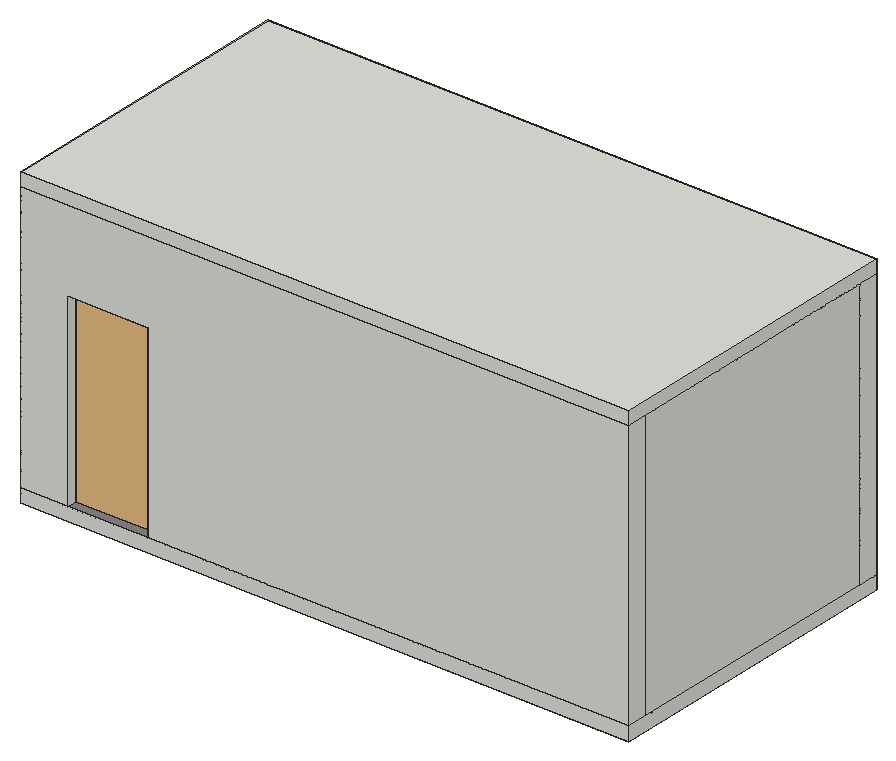
# SketchUp Ruby script. Lengths in inches.
U = 1.inch
M = Sketchup.active_model
def pt(a) = Geom::Point3d.new(a.map { |v| v * U })
def face(e, loops, mat)
  f = e.add_face(loops[0].map { |a| pt(a) })
  loops[1..].each { |l| e.add_face(l.map { |a| pt(a) }).erase! }
  f.material = f.back_material = mat if mat
  f
end
# faces: each face lists its corners as indices into pts; further lists are holes
def faces(e, pts, list, mat = nil) = list.each { |f| face(e, (f[0].is_a?(Array) ? f : [f]).map { |l| l.map { |i| pts[i] } }, mat) }
# xy, xz, yz: faces in a plane at the given z, y or x. An outline is a flat list of corners, or four numbers for a rectangle; further outlines are holes
def ring(l) = l.size == 4 ? [[l[0], l[1]], [l[2], l[1]], [l[2], l[3]], [l[0], l[3]]] : l.each_slice(2).to_a
def flat(e, list, mat, &to3) = list.each { |f| face(e, (f[0].is_a?(Array) ? f : [f]).map { |l| ring(l).map { |u, v| to3.(u, v) } }, mat) }
def xy(e, z, list, mat = nil) = flat(e, list, mat) { |x, y| [x, y, z] }
def xz(e, y, list, mat = nil) = flat(e, list, mat) { |x, z| [x, y, z] }
def yz(e, x, list, mat = nil) = flat(e, list, mat) { |y, z| [x, y, z] }
def lines(e, pts, list) = list.each { |a, b| e.add_line(pt(pts[a]), pt(pts[b])) }
# prism: a flat outline (further loops are holes) pulled along v
def prism(e, loops, v, mat = nil)
  f = face(e, loops, mat); d = Geom::Vector3d.new(v.map { |x| x * U })
  f.pushpull(f.normal.samedirection?(d) ? d.length : -d.length)
end
def box(e, o, s, mat = nil) = prism(e, [[o, [o[0] + s[0], o[1], o[2]], [o[0] + s[0], o[1] + s[1], o[2]], [o[0], o[1] + s[1], o[2]]]], [0, 0, s[2]], mat)
def at(x, y, z, deg = 0) = Geom::Transformation.translation(pt([x, y, z])) * Geom::Transformation.rotation(ORIGIN, Z_AXIS, deg.degrees)
def axes(o, x, y, z) = Geom::Transformation.new([*x, 0, *y, 0, *z, 0, *pt(o).to_a, 1])
def part(name) = M.definitions.add(name)
# library, detail: a bought-in or finely detailed component or shape, given as its bounding box
def library(name, o, s) = part(name).tap { |d| box(d.entities, o, s) }
def detail(e, o, s) = box(e.add_group.entities, o, s)
def put(e, d, t, mat = nil) = e.add_instance(d, t).tap { |i| i.material = mat if mat }
def group(e, t, mat = nil) = e.add_group.tap { |g| g.transformation = t; g.material = mat if mat }.entities
root = M.entities
M.materials.add("Generic\#1").color = [255, 244, 244]
M.materials.add("Generic\#2").color = [136, 130, 130]
M.materials.add("Tiles Simple 03 100cm").color = [137, 132, 131]
M.materials.add("Wine2").color = [0, 0, 0]
M.materials["Wine2"].alpha = 0
M.materials.add("[0130_Gainsboro]").color = [39, 45, 50]
M.materials.add("[Color F08]").color = [51, 102, 0]
M.materials.add("[Color K01]").color = [128, 97, 74]
M.materials.add("[Color M07]").color = [58, 58, 58]
M.materials.add("[Wood Veneer 01]").color = [120, 70, 37]
c1 = library("Tlon Light 450 Ceiling 152 006",[-8.86,-8.86,-3.78],[17.72,17.72,3.56])
c2 = part("Framed panel")
xy(c2.entities,0,[[0,-0.98,43.07,0],[0,0,43.07,1.4]],"[0130_Gainsboro]")
xy(c2.entities,0.3,[[0.3,-1.43,42.77,-0.98]],"[0130_Gainsboro]")
xy(c2.entities,2.95,[[2.95,-1.43,40.12,-0.63],[2.95,-0.63,40.12,0],[2.95,0,40.12,0.64],[2.95,0.64,40.12,1.4]],"[0130_Gainsboro]")
xy(c2.entities,3.54,[[3.54,-0.63,39.53,0],[3.54,0,39.53,0.64]],"[0130_Gainsboro]")
xy(c2.entities,111.8125,[[3.54,-0.63,39.53,0],[3.54,0,39.53,0.64]],"[0130_Gainsboro]")
xy(c2.entities,112.4,[[2.95,-1.43,40.12,-0.63],[2.95,-0.63,40.12,0],[2.95,0,40.12,0.64],[2.95,0.64,40.12,1.4]],"[0130_Gainsboro]")
xy(c2.entities,115.05,[[0.3,-1.43,42.77,-0.98]],"[0130_Gainsboro]")
xy(c2.entities,115.35,[[0,-0.98,43.07,0],[0,0,43.07,1.4]],"[0130_Gainsboro]")
xz(c2.entities,-1.43,[[[0.3,0.3,42.77,115.05],[2.95,2.95,40.12,112.4]]],"[0130_Gainsboro]")
xz(c2.entities,-0.98,[[[0,0,43.07,115.35],[0.3,0.3,42.77,115.05]]],"[0130_Gainsboro]")
xz(c2.entities,-0.63,[[[2.95,2.95,40.12,112.4],[3.54,3.54,39.53,111.8125]]],"[0130_Gainsboro]")
xz(c2.entities,0,[[3.54,3.54,39.53,111.8125]],"Wine2")
xz(c2.entities,0,[[[0,0,43.07,115.35],[2.95,2.95,40.12,112.4]],[[2.95,2.95,40.12,112.4],[3.54,3.54,39.53,111.8125]]],"[0130_Gainsboro]")
xz(c2.entities,0.64,[[[2.95,2.95,40.12,112.4],[3.54,3.54,39.53,111.8125]]],"[0130_Gainsboro]")
xz(c2.entities,1.4,[[[0,0,43.07,115.35],[2.95,2.95,40.12,112.4]]],"[0130_Gainsboro]")
yz(c2.entities,0,[[-0.98,0,0,115.35],[0,0,1.4,115.35]],"[0130_Gainsboro]")
yz(c2.entities,0.3,[[-1.43,0.3,-0.98,115.05]],"[0130_Gainsboro]")
yz(c2.entities,2.95,[[-1.43,2.95,-0.63,112.4],[-0.63,2.95,0,112.4],[0,2.95,0.64,112.4],[0.64,2.95,1.4,112.4]],"[0130_Gainsboro]")
yz(c2.entities,3.54,[[-0.63,3.54,0,111.8125],[0,3.54,0.64,111.8125]],"[0130_Gainsboro]")
yz(c2.entities,39.53,[[-0.63,3.54,0,111.8125],[0,3.54,0.64,111.8125]],"[0130_Gainsboro]")
yz(c2.entities,40.12,[[-1.43,2.95,-0.63,112.4],[-0.63,2.95,0,112.4],[0,2.95,0.64,112.4],[0.64,2.95,1.4,112.4]],"[0130_Gainsboro]")
yz(c2.entities,42.77,[[-1.43,0.3,-0.98,115.05]],"[0130_Gainsboro]")
yz(c2.entities,43.07,[[-0.98,0,0,115.35],[0,0,1.4,115.35]],"[0130_Gainsboro]")
c3 = part("Framed panel assembly")
put(c3.entities,c2,axes([90.57,1.43,0],[1.05148,0,0],[0,1,0],[0,0,1]))
put(c3.entities,c2,axes([0,1.43,0],[1.05148,0,0],[0,1,0],[0,0,1]))
put(c3.entities,c2,axes([45.29,1.43,0],[1.05148,0,0],[0,1,0],[0,0,1]))
c4 = library("12",[-59.59,-13.96,0.05],[132.77,19.46,130.21])
c5 = library("porta 4",[0.2,-5.42,1.33],[46.55,4.72,83.21])
c6 = library("TV Stand 144 005",[-36.8,-10.43,-0.15],[73.6,20.86,18.87])
c7 = library("Decoration 111 063",[-2.51,-1.28,-0.03],[5.02,2.53,10.66])
c8 = library("Vase Roses Red 63-02",[-2.39,-2.73,0.01],[6.39,5.25,18.18])
c9 = library("Decorative Deer 209 004",[-1.58,-4.16,0],[3.36,7.25,10.63])
c10 = library("TV Flatscreen 001",[-21.34,-8.66,-0.01],[42.68,15.88,27.55])
c11 = library("Tree Of Life Wall Art",[0,-2.17,0],[76.8125,2.17,76.8125])
c12 = library("Potted plant",[-1.15,-1.29,0],[7.65,7.78,5.89])
c13 = library("Chloe Sofa",[-57.875,-21.08,0],[115.75,42.01,35.79])
c14 = library("Vavel Meeting",[-46.89,-19.24,-0.01],[93.78,38.48,29.4])
c15 = library("Vase 007",[-9.22,-3.28,0],[11.85,5.91,21.89])
c16 = library("Armillary Sphere 37-31",[-7.11,-7.1,0],[14.21,14.18,18.13])
c17 = library("Aroma Diffuser 274 006",[-1.2,-1.19,-0.07],[2.39,2.37,8.4])
c18 = library("Carpet 274 003",[-39.19,-39.17,0],[78.4,78.37,0.4])
c19 = library("Apple 73-11",[-5.39,-5.39,0],[10.78,10.78,8.98])
c20 = library("Books 193 006",[-5.22,-3.55,0],[10.44,7.83,2.69])
c21 = library("ceiling fan",[14.63,0,0.68],[45.1,74.31,31.88])
c22 = part("fan")
p = [[217.527,-902.72,540.318],[217.529,-902.72,540.318],[217.529,-902.72,541.354],[217.527,-902.72,541.354]]
lines(c22.entities,p,[[0,1],[2,3]])
put(c22.entities,c21,at(256.45,-350.9,679.41))
c23 = library("Group\#2",[-0.5,0,0.5],[103.99,27.6,2])
c24 = library("Group\#4",[-0.5,-0.5,0],[103.99,10.6875,2])
c25 = library("Group\#5",[-0.5,-0.5,0],[150.41,81.41,2])
c26 = library("Group\#8",[0,0,0],[11.8125,120,116])
c27 = library("Group\#16",[-0.5,-0.5,-0.1],[1.5,51,0.2])
c28 = library("Group\#17",[-0.5,-0.5,0],[1.5,1,93.9375])
c29 = library("Group\#18",[-0.5,-0.5,0],[1.5,1,93.9375])
c30 = library("Group\#19",[-0.5,-0.5,-0.1],[1.5,51,0.2])
xy(root,-6,[[0,0,270.9375,138]])
xy(root,0,[[0,0,21,0,21,9,9,9,9,129,270.9375,129,270.9375,138,0,138],[57,0,270.9375,9]])
xy(root,0,[[21,0,57,0,57,9,270.9375,9,270.9375,129,9,129,9,32.0625,20.8125,32.0625,20.8125,9,21,9]],"Tiles Simple 03 100cm")
xy(root,4.46,[[18.45,129,187.89,138]])
xy(root,22.0625,[[9.5,44.37,9.9,94.37]])
xy(root,52.39,[[85.32,9,126.94,10.0625]],"[Color M07]")
xy(root,54.875,[[87.81,9.375,124.46,10.0625]],"[Color M07]")
xy(root,84,[[21,0,57,9]])
xy(root,88.84,[[18.45,129,187.89,138]])
xy(root,102.34,[[87.81,9.375,124.46,10.0625]],"[Color M07]")
xy(root,104.82,[[85.32,9,126.94,10.0625]],"[Color M07]")
xy(root,116,[[[9,9,198,129],[30.8,30.8,176.2,107.2],[9.5,44.37,9.9,94.37]],[9.5,44.37,9.9,94.37]],"Generic\#2")
xy(root,116,[[45.6,45.6,45.6,63.5,54,63.5,54,54,153,54,153,63.5,161.4,63.5,161.4,45.6],[45.6,76.31,45.6,92.4,161.4,92.4,161.4,76.31,153,76.31,153,84,54,84,54,76.31]],"[Wood Veneer 01]")
xy(root,118,[[28.8,28.8,30.8,107.2],[30.8,28.8,178.2,30.8],[176.2,30.8,178.2,107.2],[52,52,155,54],[52,54,54,63.5],
  [153,54,155,63.5],[52,76.31,54,86],[153,76.31,155,84],[54,84,155,86],[28.8,107.2,178.2,109.2]])
xy(root,120,[[0,0,0,138,270.9375,138,270.9375,129,9,129,9,9,270.9375,9,270.9375,0],[[9,9,198,129],[28.8,28.8,178.2,109.2]],[198,9,270.9375,129]])
xy(root,120,[[[28.8,28.8,178.2,109.2],[45.6,45.6,161.4,45.6,161.4,63.5,155,63.5,155,52,52,52,52,63.5,45.6,63.5],[45.6,76.31,52,76.31,52,86,155,86,155,76.31,161.4,76.31,161.4,92.4,45.6,92.4],[96.37,61.16,97.05,61.17,97.73,61.22,98.41,61.33,99.08,61.49,99.73,61.71,100.36,61.97,100.97,62.28,101.55,62.64,102.11,63.05,102.625,63.49,103.11,63.98,103.55,64.5,103.95,65.06,104.31,65.64,104.62,66.25,104.88,66.89,105.09,67.54,105.25,68.21,105.35,68.88,105.4,69.57,105.4,70.25,105.35,70.93,105.24,71.61,105.08,72.28,104.86,72.93,104.6,73.56,104.29,74.17,103.93,74.75,103.52,75.31,103.08,75.83,102.59,76.31,102.07,76.75,101.51,77.15,100.93,77.51,100.32,77.82,99.68,78.08,99.03,78.29,98.36,78.45,97.6875,78.55,97,78.61,96.32,78.6,95.63,78.55,94.96,78.4375,94.29,78.28,93.64,78.0625,93.01,77.8,92.4,77.49,91.82,77.125,91.26,76.72,90.74,76.28,90.26,75.79,89.82,75.27,89.42,74.71,89.06,74.13,88.75,73.52,88.49,72.88,88.28,72.23,88.12,71.5625,88.02,70.89,87.96,70.2,87.97,69.52,88.02,68.83,88.13,68.16,88.29,67.49,88.51,66.84,88.77,66.21,89.08,65.6,89.44,65.02,89.85,64.46,90.29,63.94,90.78,63.46,91.3,63.02,91.86,62.62,92.44,62.26,93.05,61.95,93.6875,61.69,94.34,61.48,95.01,61.32,95.68,61.22]]],"Generic\#2")
xy(root,126,[[0,0,270.9375,138]])
xz(root,0,[[0,-6,270.9375,0],[0,0,21,0,21,84,57,84,57,0,270.9375,0,270.9375,120,0,120],[0,120,270.9375,126]])
xz(root,9,[[85.32,52.39,126.94,104.82],[9,116,198,120],[198,116,270.9375,120]])
xz(root,9,[[[9,0,9,116,270.9375,116,270.9375,0,57,0,57,84,21,84,21,0],[85.32,52.39,126.94,104.82]]],"Generic\#2")
xz(root,9.375,[[87.81,54.875,124.46,102.34]],"[Color K01]")
xz(root,10.0625,[[[85.32,52.39,126.94,104.82],[87.81,54.875,124.46,102.34]]],"[Color M07]")
xz(root,30.8,[[30.8,116,176.2,118]],"Generic\#2")
xz(root,44.37,[[9.5,22.0625,9.9,116]])
xz(root,45.6,[[45.6,116,161.4,120]],"[Wood Veneer 01]")
xz(root,54,[[54,116,153,118]],"[Wood Veneer 01]")
xz(root,63.5,[[45.6,116,45.6,120,52,120,52,118,54,118,54,116],[153,116,153,118,155,118,155,120,161.4,120,161.4,116]],"[Wood Veneer 01]")
xz(root,76.31,[[45.6,116,54,116,54,118,52,118,52,120,45.6,120],[153,116,161.4,116,161.4,120,155,120,155,118,153,118]],"[Wood Veneer 01]")
xz(root,84,[[54,116,153,118]],"[Wood Veneer 01]")
xz(root,92.4,[[45.6,116,161.4,120]],"[Wood Veneer 01]")
xz(root,94.37,[[9.5,22.0625,9.9,116]])
xz(root,107.2,[[30.8,116,176.2,118]],"Generic\#2")
xz(root,129,[[9,116,198,120],[198,116,270.9375,120]])
xz(root,129,[[[9,0,270.9375,116],[18.45,4.46,187.89,88.84]]],"Generic\#2")
xz(root,138,[[0,-6,270.9375,0],[[0,0,270.9375,120],[18.45,4.46,187.89,88.84]],[0,120,270.9375,126]])
yz(root,0,[[0,-6,138,0],[0,0,138,120],[0,120,138,126]])
yz(root,9,[[[44.37,22.0625,94.37,116],[70.2,57.86,71.66,57.9375,73.11,58.12,74.55,58.4,75.96,58.78,77.34,59.26,78.6875,59.84,79.99,60.51,81.24,61.26,82.4375,62.1,83.57,63.03,84.64,64.03,85.64,65.1,86.55,66.24,87.39,67.4375,88.14,68.69,88.8,70,89.37,71.35,89.84,72.73,90.22,74.14,90.5,75.58,90.67,77.03,90.74,78.49,90.71,79.96,90.58,81.41,90.35,82.86,90.02,84.28,89.59,85.68,89.0625,87.04,88.44,88.37,87.73,89.65,86.93,90.87,86.05,92.04,85.08,93.14,84.05,94.17,82.94,95.13,81.77,96.01,80.54,96.8,79.26,97.51,77.93,98.12,76.57,98.64,75.17,99.07,73.74,99.39,72.3,99.62,70.84,99.74,69.375,99.77,67.92,99.6875,66.46,99.5,65.03,99.22,63.62,98.84,62.23,98.36,60.89,97.79,59.59,97.12,58.33,96.36,57.14,95.52,56,94.6,54.9375,93.6,53.94,92.53,53.02,91.39,52.1875,90.1875,51.4375,88.93,50.77,87.63,50.21,86.28,49.73,84.9,49.36,83.48,49.08,82.05,48.91,80.59,48.83,79.13,48.86,77.67,48.99,76.21,49.22,74.77,49.56,73.34,49.99,71.95,50.51,70.58,51.14,69.26,51.85,67.98,52.65,66.75,53.53,65.59,54.49,64.49,55.53,63.45,56.64,62.5,57.81,61.62,59.03,60.82,60.32,60.12,61.64,59.5,63.01,58.98,64.41,58.56,65.83,58.23,67.28,58.01,68.74,57.88]],[9,116,129,120]])
yz(root,9,[[9,0,129,0,129,116,94.37,116,94.37,22.0625,44.37,22.0625,44.37,116,9,116]],"Generic\#2")
yz(root,9.5,[[[44.37,22.0625,94.37,116],[70.2,57.86,71.66,57.9375,73.11,58.12,74.55,58.4,75.96,58.78,77.34,59.26,78.6875,59.84,79.99,60.51,81.24,61.26,82.4375,62.1,83.57,63.03,84.64,64.03,85.64,65.1,86.55,66.24,87.39,67.4375,88.14,68.69,88.8,70,89.37,71.35,89.84,72.73,90.22,74.14,90.5,75.58,90.67,77.03,90.74,78.49,90.71,79.96,90.58,81.41,90.35,82.86,90.02,84.28,89.59,85.68,89.0625,87.04,88.44,88.37,87.73,89.65,86.93,90.87,86.05,92.04,85.08,93.14,84.05,94.17,82.94,95.13,81.77,96.01,80.54,96.8,79.26,97.51,77.93,98.12,76.57,98.64,75.17,99.07,73.74,99.39,72.3,99.62,70.84,99.74,69.375,99.77,67.92,99.6875,66.46,99.5,65.03,99.22,63.62,98.84,62.23,98.36,60.89,97.79,59.59,97.12,58.33,96.36,57.14,95.52,56,94.6,54.9375,93.6,53.94,92.53,53.02,91.39,52.1875,90.1875,51.4375,88.93,50.77,87.63,50.21,86.28,49.73,84.9,49.36,83.48,49.08,82.05,48.91,80.59,48.83,79.13,48.86,77.67,48.99,76.21,49.22,74.77,49.56,73.34,49.99,71.95,50.51,70.58,51.14,69.26,51.85,67.98,52.65,66.75,53.53,65.59,54.49,64.49,55.53,63.45,56.64,62.5,57.81,61.62,59.03,60.82,60.32,60.12,61.64,59.5,63.01,58.98,64.41,58.56,65.83,58.23,67.28,58.01,68.74,57.88]],[70.2,57.86,71.66,57.9375,73.11,58.12,74.55,58.4,75.96,58.78,77.34,59.26,78.6875,59.84,79.99,60.51,81.24,61.26,82.4375,62.1,83.57,63.03,84.64,64.03,85.64,65.1,86.55,66.24,87.39,67.4375,88.14,68.69,88.8,70,89.37,71.35,89.84,72.73,90.22,74.14,90.5,75.58,90.67,77.03,90.74,78.49,90.71,79.96,90.58,81.41,90.35,82.86,90.02,84.28,89.59,85.68,89.0625,87.04,88.44,88.37,87.73,89.65,86.93,90.87,86.05,92.04,85.08,93.14,84.05,94.17,82.94,95.13,81.77,96.01,80.54,96.8,79.26,97.51,77.93,98.12,76.57,98.64,75.17,99.07,73.74,99.39,72.3,99.62,70.84,99.74,69.375,99.77,67.92,99.6875,66.46,99.5,65.03,99.22,63.62,98.84,62.23,98.36,60.89,97.79,59.59,97.12,58.33,96.36,57.14,95.52,56,94.6,54.9375,93.6,53.94,92.53,53.02,91.39,52.1875,90.1875,51.4375,88.93,50.77,87.63,50.21,86.28,49.73,84.9,49.36,83.48,49.08,82.05,48.91,80.59,48.83,79.13,48.86,77.67,48.99,76.21,49.22,74.77,49.56,73.34,49.99,71.95,50.51,70.58,51.14,69.26,51.85,67.98,52.65,66.75,53.53,65.59,54.49,64.49,55.53,63.45,56.64,62.5,57.81,61.62,59.03,60.82,60.32,60.12,61.64,59.5,63.01,58.98,64.41,58.56,65.83,58.23,67.28,58.01,68.74,57.88]])
yz(root,9.9,[[[44.37,22.0625,94.37,116],[70.2,57.86,68.74,57.88,67.28,58.01,65.83,58.23,64.41,58.56,63.01,58.98,61.64,59.5,60.32,60.12,59.03,60.82,57.81,61.62,56.64,62.5,55.53,63.45,54.49,64.49,53.53,65.59,52.65,66.75,51.85,67.98,51.14,69.26,50.51,70.58,49.99,71.95,49.56,73.34,49.22,74.77,48.99,76.21,48.86,77.67,48.83,79.13,48.91,80.59,49.08,82.05,49.36,83.48,49.73,84.9,50.21,86.28,50.77,87.63,51.4375,88.93,52.1875,90.1875,53.02,91.39,53.94,92.53,54.9375,93.6,56,94.6,57.14,95.52,58.33,96.36,59.59,97.12,60.89,97.79,62.23,98.36,63.62,98.84,65.03,99.22,66.46,99.5,67.92,99.6875,69.375,99.77,70.84,99.74,72.3,99.62,73.74,99.39,75.17,99.07,76.57,98.64,77.93,98.12,79.26,97.51,80.54,96.8,81.77,96.01,82.94,95.13,84.05,94.17,85.08,93.14,86.05,92.04,86.93,90.87,87.73,89.65,88.44,88.37,89.0625,87.04,89.59,85.68,90.02,84.28,90.35,82.86,90.58,81.41,90.71,79.96,90.74,78.49,90.67,77.03,90.5,75.58,90.22,74.14,89.84,72.73,89.37,71.35,88.8,70,88.14,68.69,87.39,67.4375,86.55,66.24,85.64,65.1,84.64,64.03,83.57,63.03,82.4375,62.1,81.24,61.26,79.99,60.51,78.6875,59.84,77.34,59.26,75.96,58.78,74.55,58.4,73.11,58.12,71.66,57.9375]]],"Generic\#1")
yz(root,18.45,[[129,4.46,138,88.84]])
yz(root,21,[[0,0,9,84]])
yz(root,30.8,[[30.8,116,107.2,118]],"Generic\#2")
yz(root,45.6,[[45.6,116,63.5,120],[76.31,116,92.4,120]],"[Wood Veneer 01]")
yz(root,54,[[54,116,63.5,118],[76.31,116,84,118]],"[Wood Veneer 01]")
yz(root,57,[[0,0,9,84]])
yz(root,85.32,[[9,52.39,10.0625,104.82]],"[Color M07]")
yz(root,87.81,[[9.375,54.875,10.0625,102.34]],"[Color M07]")
yz(root,124.46,[[9.375,54.875,10.0625,102.34]],"[Color M07]")
yz(root,126.94,[[9,52.39,10.0625,104.82]],"[Color M07]")
yz(root,153,[[54,116,63.5,118],[76.31,116,84,118]],"[Wood Veneer 01]")
yz(root,161.4,[[45.6,116,63.5,120],[76.31,116,92.4,120]],"[Wood Veneer 01]")
yz(root,176.2,[[30.8,116,107.2,118]],"Generic\#2")
yz(root,187.89,[[129,4.46,138,88.84]])
yz(root,198,[[9,116,129,120]])
yz(root,270.9375,[[0,-6,138,0],[0,0,9,120],[9,0,129,120],[129,0,138,120],[0,120,138,126]])
p = [[9.5,68.74,57.88],[9.5,67.28,58.01],[9,67.28,58.01],[9,68.74,57.88],[9.9,67.28,58.01],[9.9,68.74,57.88],
  [9.5,70.2,57.86],[9,70.2,57.86],[9.9,70.2,57.86],[9.5,71.66,57.9375],[9,71.66,57.9375],[9.9,71.66,57.9375],
  [9.5,73.11,58.12],[9,73.11,58.12],[9.9,73.11,58.12],[9.5,65.83,58.23],[9,65.83,58.23],[9.9,65.83,58.23],
  [9.5,74.55,58.4],[9,74.55,58.4],[9.9,74.55,58.4],[9.5,64.41,58.56],[9,64.41,58.56],[9.9,64.41,58.56],
  [9.5,75.96,58.78],[9,75.96,58.78],[9.9,75.96,58.78],[9.5,63.01,58.98],[9,63.01,58.98],[9.9,63.01,58.98],
  [9.5,77.34,59.26],[9,77.34,59.26],[9.9,77.34,59.26],[9.5,61.64,59.5],[9,61.64,59.5],[9.9,61.64,59.5],
  [9.5,78.6875,59.84],[9,78.6875,59.84],[9.9,78.6875,59.84],[9.5,60.32,60.12],[9,60.32,60.12],[9.9,60.32,60.12],
  [9.5,79.99,60.51],[9,79.99,60.51],[9.9,79.99,60.51],[9.5,59.03,60.82],[9,59.03,60.82],[9.9,59.03,60.82],
  [9.5,81.24,61.26],[9,81.24,61.26],[9.9,81.24,61.26],[9.5,57.81,61.62],[9,57.81,61.62],[9.9,57.81,61.62],
  [9.5,82.4375,62.1],[9,82.4375,62.1],[9.9,82.4375,62.1],[9.5,56.64,62.5],[9,56.64,62.5],[9.9,56.64,62.5],
  [9.5,83.57,63.03],[9,83.57,63.03],[9.9,83.57,63.03],[9.5,55.53,63.45],[9,55.53,63.45],[9.9,55.53,63.45],
  [9.5,84.64,64.03],[9,84.64,64.03],[9.9,84.64,64.03],[9.5,54.49,64.49],[9,54.49,64.49],[9.9,54.49,64.49],
  [9.5,85.64,65.1],[9,85.64,65.1],[9.9,85.64,65.1],[9.5,53.53,65.59],[9,53.53,65.59],[9.9,53.53,65.59],
  [9.5,86.55,66.24],[9,86.55,66.24],[9.9,86.55,66.24],[9.5,52.65,66.75],[9,52.65,66.75],[9.9,52.65,66.75],
  [9.5,87.39,67.4375],[9,87.39,67.4375],[9.9,87.39,67.4375],[9.5,51.85,67.98],[9,51.85,67.98],[9.9,51.85,67.98],
  [9.5,88.14,68.69],[9,88.14,68.69],[9.9,88.14,68.69],[9.5,51.14,69.26],[9,51.14,69.26],[9.9,51.14,69.26],
  [9.5,88.8,70],[9,88.8,70],[9.9,88.8,70],[9.5,50.51,70.58],[9,50.51,70.58],[9.9,50.51,70.58],
  [9.5,89.37,71.35],[9,89.37,71.35],[9.9,89.37,71.35],[9.5,49.99,71.95],[9,49.99,71.95],[9.9,49.99,71.95],
  [9.5,89.84,72.73],[9,89.84,72.73],[9.9,89.84,72.73],[9.5,49.56,73.34],[9,49.56,73.34],[9.9,49.56,73.34],
  [9.5,90.22,74.14],[9,90.22,74.14],[9.9,90.22,74.14],[9.5,49.22,74.77],[9,49.22,74.77],[9.9,49.22,74.77],
  [9.5,90.5,75.58],[9,90.5,75.58],[9.9,90.5,75.58],[9.5,48.99,76.21],[9,48.99,76.21],[9.9,48.99,76.21],
  [9.5,90.67,77.03],[9,90.67,77.03],[9.9,90.67,77.03],[9.5,48.86,77.67],[9,48.86,77.67],[9.9,48.86,77.67],
  [9.5,90.74,78.49],[9,90.74,78.49],[9.9,90.74,78.49],[9.5,48.83,79.13],[9,48.83,79.13],[9.9,48.83,79.13],
  [9.5,90.71,79.96],[9,90.71,79.96],[9.9,90.71,79.96],[9.5,48.91,80.59],[9,48.91,80.59],[9.9,48.91,80.59],
  [9.5,90.58,81.41],[9,90.58,81.41],[9.9,90.58,81.41],[9.5,49.08,82.05],[9,49.08,82.05],[9.9,49.08,82.05],
  [9.5,90.35,82.86],[9,90.35,82.86],[9.9,90.35,82.86],[9.5,49.36,83.48],[9,49.36,83.48],[9.9,49.36,83.48],
  [9.5,90.02,84.28],[9,90.02,84.28],[9.9,90.02,84.28],[9.5,49.73,84.9],[9,49.73,84.9],[9.9,49.73,84.9],
  [9.5,89.59,85.68],[9,89.59,85.68],[9.9,89.59,85.68],[9.5,50.21,86.28],[9,50.21,86.28],[9.9,50.21,86.28],
  [9.5,89.0625,87.04],[9,89.0625,87.04],[9.9,89.0625,87.04],[9.5,50.77,87.63],[9,50.77,87.63],[9.9,50.77,87.63],
  [9.5,88.44,88.37],[9,88.44,88.37],[9.9,88.44,88.37],[9.5,51.4375,88.93],[9,51.4375,88.93],[9.9,51.4375,88.93],
  [9.5,87.73,89.65],[9,87.73,89.65],[9.9,87.73,89.65],[9.5,52.1875,90.1875],[9,52.1875,90.1875],[9.9,52.1875,90.1875],
  [9.5,86.93,90.87],[9,86.93,90.87],[9.9,86.93,90.87],[9.5,53.02,91.39],[9,53.02,91.39],[9.9,53.02,91.39],
  [9.5,86.05,92.04],[9,86.05,92.04],[9.9,86.05,92.04],[9.5,53.94,92.53],[9,53.94,92.53],[9.9,53.94,92.53],
  [9.5,85.08,93.14],[9,85.08,93.14],[9.9,85.08,93.14],[9.5,54.9375,93.6],[9,54.9375,93.6],[9.9,54.9375,93.6],
  [9.5,84.05,94.17],[9,84.05,94.17],[9.9,84.05,94.17],[9.5,56,94.6],[9,56,94.6],[9.9,56,94.6],
  [9.5,82.94,95.13],[9,82.94,95.13],[9.9,82.94,95.13],[9.5,57.14,95.52],[9,57.14,95.52],[9.9,57.14,95.52],
  [9.5,81.77,96.01],[9,81.77,96.01],[9.9,81.77,96.01],[9.5,58.33,96.36],[9,58.33,96.36],[9.9,58.33,96.36],
  [9.5,80.54,96.8],[9,80.54,96.8],[9.9,80.54,96.8],[9.5,59.59,97.12],[9,59.59,97.12],[9.9,59.59,97.12],
  [9.5,79.26,97.51],[9,79.26,97.51],[9.9,79.26,97.51],[9.5,60.89,97.79],[9,60.89,97.79],[9.9,60.89,97.79],
  [9.5,77.93,98.12],[9,77.93,98.12],[9.9,77.93,98.12],[9.5,62.23,98.36],[9,62.23,98.36],[9.9,62.23,98.36],
  [9.5,76.57,98.64],[9,76.57,98.64],[9.9,76.57,98.64],[9.5,63.62,98.84],[9,63.62,98.84],[9.9,63.62,98.84],
  [9.5,75.17,99.07],[9,75.17,99.07],[9.9,75.17,99.07],[9.5,65.03,99.22],[9,65.03,99.22],[9.9,65.03,99.22],
  [9.5,73.74,99.39],[9,73.74,99.39],[9.9,73.74,99.39],[9.5,66.46,99.5],[9,66.46,99.5],[9.9,66.46,99.5],
  [9.5,72.3,99.62],[9,72.3,99.62],[9.9,72.3,99.62],[9.5,67.92,99.6875],[9,67.92,99.6875],[9.9,67.92,99.6875],
  [9.5,70.84,99.74],[9,70.84,99.74],[9.9,70.84,99.74],[9.5,69.375,99.77],[9,69.375,99.77],[9.9,69.375,99.77],
  [10,89.53,78.8125],[10,89.54,78.59],[10,89.53,78.375]]
faces(root,p,[[0,1,2,3],[0,1,4,5],[6,0,3,7],[6,0,5,8],[9,6,7,10],[9,6,8,11],[12,9,10,13],[12,9,11,14],
  [1,15,16,2],[1,15,17,4],[18,12,13,19],[18,12,14,20],[15,21,22,16],[15,21,23,17],[24,18,19,25],[24,18,20,26],
  [21,27,28,22],[21,27,29,23],[30,24,25,31],[30,24,26,32],[27,33,34,28],[27,33,35,29],[36,30,31,37],[36,30,32,38],
  [33,39,40,34],[33,39,41,35],[42,36,37,43],[42,36,38,44],[39,45,46,40],[39,45,47,41],[48,42,43,49],[48,42,44,50],
  [45,51,52,46],[45,51,53,47],[54,48,49,55],[54,48,50,56],[51,57,58,52],[51,57,59,53],[60,54,55,61],[60,54,56,62],
  [57,63,64,58],[57,63,65,59],[66,60,61,67],[66,60,62,68],[63,69,70,64],[63,69,71,65],[72,66,67,73],[72,66,68,74],
  [69,75,76,70],[69,75,77,71],[78,72,73,79],[78,72,74,80],[75,81,82,76],[75,81,83,77],[84,78,79,85],[84,78,80,86],
  [81,87,88,82],[81,87,89,83],[90,84,85,91],[90,84,86,92],[87,93,94,88],[87,93,95,89],[96,90,91,97],[96,90,92,98],
  [93,99,100,94],[93,99,101,95],[102,96,97,103],[102,96,98,104],[99,105,106,100],[99,105,107,101],[108,102,103,109],[108,102,104,110],
  [105,111,112,106],[105,111,113,107],[114,108,109,115],[114,108,110,116],[111,117,118,112],[111,117,119,113],[120,114,115,121],[120,114,116,122],
  [117,123,124,118],[117,123,125,119],[126,120,121,127],[126,120,122,128],[123,129,130,124],[123,129,131,125],[132,126,127,133],[132,126,128,134],
  [129,135,136,130],[129,135,137,131],[138,132,133,139],[138,132,134,140],[135,141,142,136],[135,141,143,137],[144,138,139,145],[144,138,140,146],
  [141,147,148,142],[141,147,149,143],[150,144,145,151],[150,144,146,152],[147,153,154,148],[147,153,155,149],[156,150,151,157],[156,150,152,158],
  [153,159,160,154],[153,159,161,155],[162,156,157,163],[162,156,158,164],[159,165,166,160],[159,165,167,161],[168,162,163,169],[168,162,164,170],
  [165,171,172,166],[165,171,173,167],[174,168,169,175],[174,168,170,176],[171,177,178,172],[171,177,179,173],[180,174,175,181],[180,174,176,182],
  [177,183,184,178],[177,183,185,179],[186,180,181,187],[186,180,182,188],[183,189,190,184],[183,189,191,185],[192,186,187,193],[192,186,188,194],
  [189,195,196,190],[189,195,197,191],[198,192,193,199],[198,192,194,200],[195,201,202,196],[195,201,203,197],[204,198,199,205],[204,198,200,206],
  [201,207,208,202],[201,207,209,203],[210,204,205,211],[210,204,206,212],[207,213,214,208],[207,213,215,209],[216,210,211,217],[216,210,212,218],
  [213,219,220,214],[213,219,221,215],[222,216,217,223],[222,216,218,224],[219,225,226,220],[219,225,227,221],[228,222,223,229],[228,222,224,230],
  [225,231,232,226],[225,231,233,227],[234,228,229,235],[234,228,230,236],[231,237,238,232],[231,237,239,233],[240,234,235,241],[240,234,236,242],
  [237,243,244,238],[237,243,245,239],[246,240,241,247],[246,240,242,248],[243,249,250,244],[243,249,251,245],[252,246,247,253],[252,246,248,254],
  [249,255,256,250],[249,255,257,251],[258,252,253,259],[258,252,254,260],[255,261,262,256],[255,261,263,257],[264,258,259,265],[264,258,260,266],
  [261,267,268,262],[261,267,269,263],[267,264,265,268],[267,264,266,269]])
lines(root,p,[[270,271],[272,271]])
detail(root,[85.97,59.17,116],[21.43,21.43,4])
put(root,c1,axes([29.57,18.92,116.72],[0.33758,0.0388,-0.01151],[-0.0388,0.33778,0.00066],[0.01151,0.00066,0.3398]))
put(root,c1,axes([29.57,115.98,116.72],[0.33758,0.0388,-0.01151],[-0.0388,0.33778,0.00066],[0.01151,0.00066,0.3398]))
put(root,c1,axes([62.94,18.92,116.72],[0.33758,0.0388,-0.01151],[-0.0388,0.33778,0.00066],[0.01151,0.00066,0.3398]))
put(root,c1,axes([62.94,115.98,116.72],[0.33758,0.0388,-0.01151],[-0.0388,0.33778,0.00066],[0.01151,0.00066,0.3398]))
put(root,c1,axes([96.32,18.92,116.72],[0.33758,0.0388,-0.01151],[-0.0388,0.33778,0.00066],[0.01151,0.00066,0.3398]))
put(root,c1,axes([96.32,115.98,116.72],[0.33758,0.0388,-0.01151],[-0.0388,0.33778,0.00066],[0.01151,0.00066,0.3398]))
put(root,c1,axes([129.69,18.92,116.72],[0.33758,0.0388,-0.01151],[-0.0388,0.33778,0.00066],[0.01151,0.00066,0.3398]))
put(root,c1,axes([129.69,115.98,116.72],[0.33758,0.0388,-0.01151],[-0.0388,0.33778,0.00066],[0.01151,0.00066,0.3398]))
put(root,c1,axes([163.07,18.92,116.72],[0.33758,0.0388,-0.01151],[-0.0388,0.33778,0.00066],[0.01151,0.00066,0.3398]))
put(root,c1,axes([163.07,115.98,116.72],[0.33758,0.0388,-0.01151],[-0.0388,0.33778,0.00066],[0.01151,0.00066,0.3398]))
put(root,c3,axes([18.05,131.8,4.24],[1.25,0,0],[0,1,0],[0,0,0.74]))
put(root,c4,axes([91.08,132.9375,-2.82],[1.46112,0,0],[0,1,0],[0,0,0.94288]))
put(root,c5,axes([57.16,3.8,-1.35],[-0.77339,0,0],[0,-1,0],[0,0,1.0096]))
put(root,c6,axes([14.91,69.13,0.15],[0,1,0],[-0.56635,0,0],[0,0,1]))
put(root,c7,at(16.22,20.91,19.75,90))
put(root,c8,axes([18.27,19.73,59.41],[1,0,0],[0,1,0],[0,0,0.688]))
put(root,c9,at(15.21,19.17,39.58,90))
put(root,c9,at(16.65,20.92,2.29,90))
put(root,c9,at(15.21,116.3,40.19,90))
put(root,c8,axes([18.27,116.86,59.41],[1,0,0],[0,1,0],[0,0,0.688]))
put(root,c7,at(16.22,118.03,19.75,90))
put(root,c9,at(16.65,118.04,3.19,90))
put(root,c10,axes([10.82,69.46,18.89],[0,1.2971,0],[-1,0,0],[0,0,1.5515]))
put(root,c11,axes([9.5,58.33,62.22],[0,0.3038,0],[-0.0682,0,0],[0,0,0.434]),"[Color F08]")
put(root,c12,at(14.86,33.3,18.87))
put(root,c12,at(15.32,96.85,18.87))
put(root,c13,axes([129.6,23.71,0],[-1.11969,0,0],[0,-0.70297,0],[0,0,0.9516]))
put(root,c13,axes([126.32,112.87,0],[1.11969,0,0],[0,0.70297,0],[0,0,0.9516]))
put(root,c14,axes([107.875,66.42,0.59],[1,0,0],[0,0.65,0],[0,0,0.7]))
put(root,c15,at(112.625,68.59,21.16))
put(root,c15,at(17.55,41.22,18.87))
put(root,c16,axes([16.34,20.3,99.06],[0.63,0,0],[0,0.63,0],[0,0,0.63]))
put(root,c16,axes([16.34,117.73,99.06],[0.63,0,0],[0,0.63,0],[0,0,0.63]))
put(root,c17,axes([18.49,21.77,79.26],[1,0,0],[0,1.44,0],[0,0,1.3216]))
put(root,c17,axes([17.83,118.47,79.33],[1,0,0],[0,1.44,0],[0,0,1.3216]))
put(root,c18,axes([111.52,67.84,0],[1.134,0,0],[0,0.63,0],[0,0,2.7153]))
put(root,c19,at(101.6,68.73,21.16))
put(root,c20,at(124.45,67.81,21.16))
put(root,c22,at(-196.78,366.56,-591.97))
put(root,c23,axes([52,79.11,120.5],[1,0,0],[0,-1,0],[0,0,-1]))
put(root,c24,axes([52,86,120],[1,0,0],[0,-1,0],[0,0,-1]))
put(root,c25,axes([28.8,109.2,120],[1,0,0],[0,-1,0],[0,0,-1]))
put(root,c26,at(9,9,0),"[Wood Veneer 01]")
g1 = group(root,at(9,33.37,19.0625),"[Color M07]")
box(g1,[0,71.13,0],[0.9,1.44,96.9375])
box(g1,[0,-1.31,0],[0.9,1.44,96.9375])
box(g1,[0,0.25,0],[0.9,1.44,96.9375])
box(g1,[0,1.82,0],[0.9,1.43,96.9375])
box(g1,[0,3.38,0],[0.9,1.44,96.9375])
box(g1,[0,4.94,0],[0.9,1.44,96.9375])
box(g1,[0,6.5,0],[0.9,1.44,96.9375])
box(g1,[0,69.63,0],[0.9,1.44,96.9375])
box(g1,[0,68.13,0],[0.9,1.44,96.9375])
box(g1,[0,66.63,0],[0.9,1.44,96.9375])
box(g1,[0,65.13,0],[0.9,1.44,96.9375])
box(g1,[0,63.63,0],[0.9,1.44,96.9375])
put(root,c27,at(9,44.37,116))
put(root,c28,at(9,44.37,22.0625))
put(root,c29,at(9,94.37,22.0625))
put(root,c30,at(9,44.37,22.0625))
